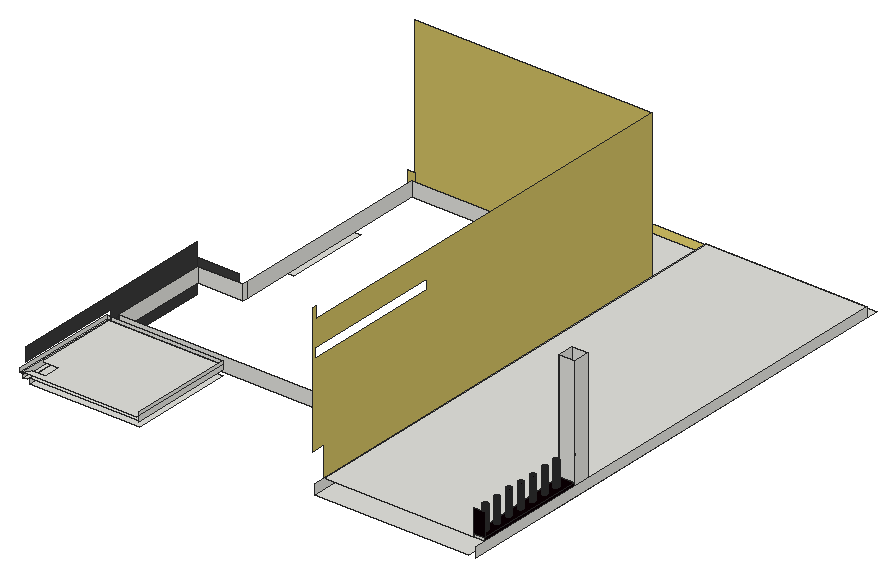
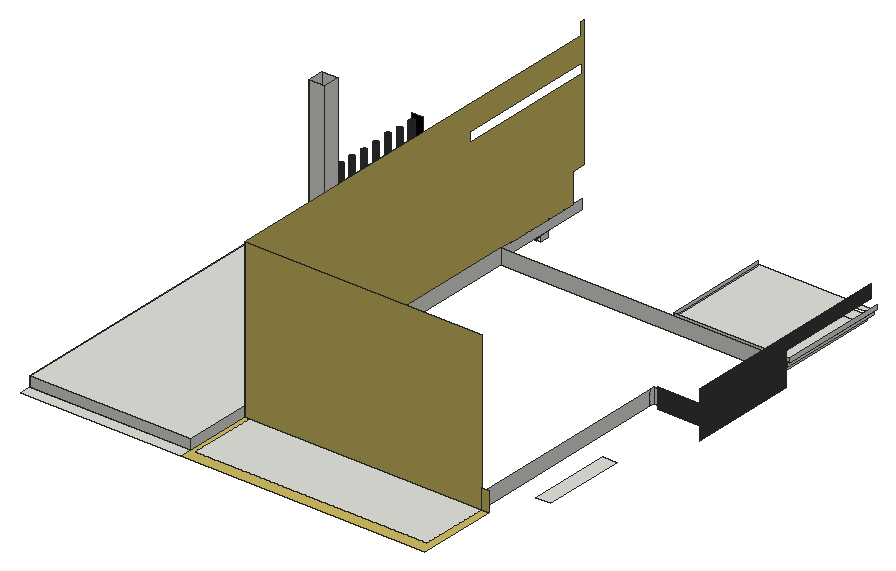
# SketchUp Ruby script. Lengths in inches.
U = 1.inch
M = Sketchup.active_model
def pt(a) = Geom::Point3d.new(a.map { |v| v * U })
def face(e, loops, mat)
  f = e.add_face(loops[0].map { |a| pt(a) })
  loops[1..].each { |l| e.add_face(l.map { |a| pt(a) }).erase! }
  f.material = f.back_material = mat if mat
  f
end
# faces: each face lists its corners as indices into pts; further lists are holes
def faces(e, pts, list, mat = nil) = list.each { |f| face(e, (f[0].is_a?(Array) ? f : [f]).map { |l| l.map { |i| pts[i] } }, mat) }
# xy, xz, yz: faces in a plane at the given z, y or x. An outline is a flat list of corners, or four numbers for a rectangle; further outlines are holes
def ring(l) = l.size == 4 ? [[l[0], l[1]], [l[2], l[1]], [l[2], l[3]], [l[0], l[3]]] : l.each_slice(2).to_a
def flat(e, list, mat, &to3) = list.each { |f| face(e, (f[0].is_a?(Array) ? f : [f]).map { |l| ring(l).map { |u, v| to3.(u, v) } }, mat) }
def xy(e, z, list, mat = nil) = flat(e, list, mat) { |x, y| [x, y, z] }
def xz(e, y, list, mat = nil) = flat(e, list, mat) { |x, z| [x, y, z] }
def yz(e, x, list, mat = nil) = flat(e, list, mat) { |y, z| [x, y, z] }
def lines(e, pts, list) = list.each { |a, b| e.add_line(pt(pts[a]), pt(pts[b])) }
# prism: a flat outline (further loops are holes) pulled along v
def prism(e, loops, v, mat = nil)
  f = face(e, loops, mat); d = Geom::Vector3d.new(v.map { |x| x * U })
  f.pushpull(f.normal.samedirection?(d) ? d.length : -d.length)
end
def box(e, o, s, mat = nil) = prism(e, [[o, [o[0] + s[0], o[1], o[2]], [o[0] + s[0], o[1] + s[1], o[2]], [o[0], o[1] + s[1], o[2]]]], [0, 0, s[2]], mat)
def at(x, y, z, deg = 0) = Geom::Transformation.translation(pt([x, y, z])) * Geom::Transformation.rotation(ORIGIN, Z_AXIS, deg.degrees)
def axes(o, x, y, z) = Geom::Transformation.new([*x, 0, *y, 0, *z, 0, *pt(o).to_a, 1])
def part(name) = M.definitions.add(name)
# library, detail: a bought-in or finely detailed component or shape, given as its bounding box
def library(name, o, s) = part(name).tap { |d| box(d.entities, o, s) }
def detail(e, o, s) = box(e.add_group.entities, o, s)
def put(e, d, t, mat = nil) = e.add_instance(d, t).tap { |i| i.material = mat if mat }
def group(e, t, mat = nil) = e.add_group.tap { |g| g.transformation = t; g.material = mat if mat }.entities
root = M.entities
M.materials.add("[Color D05]").color = [208, 191, 99]
M.materials.add("[Color M07]").color = [58, 58, 58]
M.materials.add("[Metal Seamed]").color = [11, 0, 4]
xy(root,386.54,[[389.45,106.41,450.64,113.66]])
xy(root,386.56,[[384.5,104.22,390.89,113.66],[450.58,104.22,454.38,113.66]])
xy(root,386.84,[[390.89,104.22,450.58,113.66]])
xy(root,392.6,[[55.1875,410.35,72.6875,511.06]])
xy(root,393.87,[[384.5,104.22,454.38,113.66]])
xy(root,408,[[24.25,69.47,158,195.41],[369.3125,70.97,369.3125,113.66,471.3125,113.66,471.3125,195.41,564.5,195.41,564.5,84.18,555.7,84.18,555.7,70.97],[369.3125,113.66,465.3125,119.66],[465.3125,113.66,465.3125,195.41,369.3125,195.41,369.3125,664.97,555.3125,664.97,555.3125,195.41,471.3125,195.41,471.3125,113.66],[369.3125,119.66,465.3125,195.41],
  [555.3125,195.41,564.3125,664.97],[564.3125,195.41,564.5,664.97],[81.6875,582.91,363.3125,665.75],[369.3125,664.97,564.3125,679.25]])
xy(root,408,[[72.6875,582.91,81.6875,582.91,81.6875,665.75,363.3125,665.75,363.3125,582.91,369.3125,582.91,369.3125,679.25,72.6875,679.25]],"[Color D05]")
xy(root,414.75,[[19.4375,65.66,19.4375,195.41,24.25,195.41,24.25,67.28,21.75,67.28,21.75,65.66],[24.25,69.47,158,195.41]])
xy(root,420,[[369.3125,84.66,550.8125,84.66,545.3,221.65,545.3,240.85,564.5,240.85,564.5,664.97,369.3125,664.97],[550.8125,84.66,545.3,221.65,564.5,221.65,564.5,84.66],[545.3,221.65,564.5,240.85]])
xy(root,420.5,[[17.375,63.91,17.375,195.41,19.4375,195.41,19.4375,65.66,21.75,65.66,21.75,63.91],[19.4375,65.66,158,65.66,158,195.41,19.4375,195.41,19.4375,92.83,41.19,92.83,41.19,73.08,24.07,73.08,24.07,70.02,19.4375,70.02]])
xy(root,423.375,[[554.92,94.18,554.11,94.29,553.36,94.6,552.71,95.1,552.21,95.75,551.9,96.5,551.79,97.31,551.9,98.12,552.21,98.87,552.71,99.52,553.36,100.01,554.11,100.33,554.92,100.43,555.73,100.33,556.48,100.01,557.13,99.52,557.625,98.87,557.9375,98.12,558.04,97.31,557.9375,96.5,557.625,95.75,557.13,95.1,556.48,94.6,555.73,94.29],[554.92,130.31,554.11,130.41,553.36,130.73,552.71,131.22,552.21,131.87,551.9,132.625,551.79,133.43,551.9,134.24,552.21,135,552.71,135.64,553.36,136.14,554.11,136.45,554.92,136.56,555.73,136.45,556.48,136.14,557.13,135.64,557.625,135,557.9375,134.24,558.04,133.43,557.9375,132.625,557.625,131.87,557.13,131.22,556.48,130.73,555.73,130.41],[554.92,148.37,554.11,148.48,553.36,148.79,552.71,149.29,552.21,149.93,551.9,150.6875,551.79,151.5,551.9,152.3,552.21,153.06,552.71,153.71,553.36,154.2,554.11,154.51,554.92,154.62,555.73,154.51,556.48,154.2,557.13,153.71,557.625,153.06,557.9375,152.3,558.04,151.5,557.9375,150.6875,557.625,149.93,557.13,149.29,556.48,148.79,555.73,148.48],[554.92,166.43,554.11,166.54,553.36,166.85,552.71,167.35,552.21,168,551.9,168.75,551.79,169.56,551.9,170.37,552.21,171.12,552.71,171.77,553.36,172.26,554.11,172.58,554.92,172.68,555.73,172.58,556.48,172.26,557.13,171.77,557.625,171.12,557.9375,170.37,558.04,169.56,557.9375,168.75,557.625,168,557.13,167.35,556.48,166.85,555.73,166.54],[554.92,184.5,554.11,184.6,553.36,184.91,552.71,185.41,552.21,186.06,551.9,186.8125,551.79,187.62,551.9,188.43,552.21,189.18,552.71,189.83,553.36,190.33,554.11,190.64,554.92,190.75,555.73,190.64,556.48,190.33,557.13,189.83,557.625,189.18,557.9375,188.43,558.04,187.62,557.9375,186.8125,557.625,186.06,557.13,185.41,556.48,184.91,555.73,184.6],
  [554.92,201.87,554.11,201.98,553.36,202.29,552.71,202.79,552.21,203.43,551.9,204.1875,551.79,205,551.9,205.8,552.21,206.56,552.71,207.21,553.36,207.7,554.11,208.01,554.92,208.12,555.73,208.01,556.48,207.7,557.13,207.21,557.625,206.56,557.9375,205.8,558.04,205,557.9375,204.1875,557.625,203.43,557.13,202.79,556.48,202.29,555.73,201.98]])
xy(root,423.375,[[[550.8125,84.66,564.5,84.66,564.5,221.65,545.3,221.65],[554.92,94.18,554.11,94.29,553.36,94.6,552.71,95.1,552.21,95.75,551.9,96.5,551.79,97.31,551.9,98.12,552.21,98.87,552.71,99.52,553.36,100.01,554.11,100.33,554.92,100.43,555.73,100.33,556.48,100.01,557.13,99.52,557.625,98.87,557.9375,98.12,558.04,97.31,557.9375,96.5,557.625,95.75,557.13,95.1,556.48,94.6,555.73,94.29],[554.92,112.25,554.11,112.35,553.36,112.66,552.71,113.16,552.21,113.81,551.9,114.5625,551.79,115.37,551.9,116.18,552.21,116.93,552.71,117.58,553.36,118.08,554.11,118.39,554.92,118.5,555.73,118.39,556.48,118.08,557.13,117.58,557.625,116.93,557.9375,116.18,558.04,115.37,557.9375,114.5625,557.625,113.81,557.13,113.16,556.48,112.66,555.73,112.35],[554.92,130.31,554.11,130.41,553.36,130.73,552.71,131.22,552.21,131.87,551.9,132.625,551.79,133.43,551.9,134.24,552.21,135,552.71,135.64,553.36,136.14,554.11,136.45,554.92,136.56,555.73,136.45,556.48,136.14,557.13,135.64,557.625,135,557.9375,134.24,558.04,133.43,557.9375,132.625,557.625,131.87,557.13,131.22,556.48,130.73,555.73,130.41],[554.92,148.37,554.11,148.48,553.36,148.79,552.71,149.29,552.21,149.93,551.9,150.6875,551.79,151.5,551.9,152.3,552.21,153.06,552.71,153.71,553.36,154.2,554.11,154.51,554.92,154.62,555.73,154.51,556.48,154.2,557.13,153.71,557.625,153.06,557.9375,152.3,558.04,151.5,557.9375,150.6875,557.625,149.93,557.13,149.29,556.48,148.79,555.73,148.48],[554.92,166.43,554.11,166.54,553.36,166.85,552.71,167.35,552.21,168,551.9,168.75,551.79,169.56,551.9,170.37,552.21,171.12,552.71,171.77,553.36,172.26,554.11,172.58,554.92,172.68,555.73,172.58,556.48,172.26,557.13,171.77,557.625,171.12,557.9375,170.37,558.04,169.56,557.9375,168.75,557.625,168,557.13,167.35,556.48,166.85,555.73,166.54],[554.92,184.5,554.11,184.6,553.36,184.91,552.71,185.41,552.21,186.06,551.9,186.8125,551.79,187.62,551.9,188.43,552.21,189.18,552.71,189.83,553.36,190.33,554.11,190.64,554.92,190.75,555.73,190.64,556.48,190.33,557.13,189.83,557.625,189.18,557.9375,188.43,558.04,187.62,557.9375,186.8125,557.625,186.06,557.13,185.41,556.48,184.91,555.73,184.6],[554.92,201.87,554.11,201.98,553.36,202.29,552.71,202.79,552.21,203.43,551.9,204.1875,551.79,205,551.9,205.8,552.21,206.56,552.71,207.21,553.36,207.7,554.11,208.01,554.92,208.12,555.73,208.01,556.48,207.7,557.13,207.21,557.625,206.56,557.9375,205.8,558.04,205,557.9375,204.1875,557.625,203.43,557.13,202.79,556.48,202.29,555.73,201.98]]],"[Metal Seamed]")
xz(root,84.66,[[550.8125,420,564.5,423.375]])
xz(root,84.66,[[550.8125,423.375,564.5,451.5625]],"[Metal Seamed]")
xz(root,104.22,[[384.5,386.56,390.89,386.56,390.89,386.84,450.58,386.84,450.58,386.56,454.38,386.56,454.38,393.87,384.5,393.87]])
xz(root,195.41,[[21.75,408,24.25,414.75],[19.4375,414.75,21.75,420.5],[21.75,414.75,158,420.5],[17.375,420.5,21.75,425],[21.75,420.5,158,425]])
xz(root,201.41,[[26.75,408,363.3125,426]])
xz(root,221.65,[[545.3,420,564.5,423.375],[545.3,423.375,564.5,423.375,564.5,451.5625,563.5625,451.5625,563.5625,456,564.5,456,564.5,555.625,545.3,555.625]])
xz(root,240.85,[[545.3,420,564.5,555.625]])
xz(root,320.85,[[26.75,408,81.6875,426]])
xz(root,326.53,[[21.75,408,72.6875,432]],"[Color M07]")
xz(root,578.04,[[81.6875,408,363.3125,426]])
xz(root,582.91,[[72.6875,408,81.6875,432],[81.6875,408,369.3125,598.25]],"[Color D05]")
xz(root,664.97,[[369.3125,408,564.5,420]])
yz(root,17.375,[[63.91,420.5,195.41,425]])
yz(root,19.4375,[[65.66,414.75,195.41,420.5]])
yz(root,21.75,[[195.41,391.47,326.53,420.03],[195.41,420.03,195.41,432,67.28,432,67.28,448.0625,326.53,448.0625,326.53,420.03]],"[Color M07]")
yz(root,24.25,[[69.47,408,195.41,414.75]])
yz(root,26.75,[[201.41,408,320.85,426]])
yz(root,81.6875,[[320.85,408,326.53,426],[326.53,408,578.04,426]])
yz(root,158,[[67.28,414.75,195.41,420.5],[67.28,420.5,195.41,425]])
yz(root,363.3125,[[201.41,408,578.04,426]])
yz(root,369.3125,[[70.97,408,582.91,420],[582.91,408,664.97,420]])
yz(root,369.3125,[[[84.66,420,582.91,420,582.91,598.25,72.19,598.25,72.19,612.8125,67.28,612.8125,67.28,456,84.66,456],[70.97,555.625,240.85,567.625]]],"[Color D05]")
yz(root,384.5,[[104.22,386.56,113.66,393.87]])
yz(root,390.89,[[104.22,386.56,113.66,386.84]])
yz(root,450.58,[[104.22,386.56,113.66,386.84]])
yz(root,454.38,[[104.22,386.56,113.66,393.87]])
yz(root,545.3,[[221.65,420,240.85,555.625]])
yz(root,564.5,[[70.97,408,664.97,420],[221.65,420,240.85,420,240.85,555.625,221.65,555.625,221.65,456,222.34,456,222.34,451.5625,221.65,451.5625]])
yz(root,564.5,[[84.66,420,221.65,423.375]],"[Metal Seamed]")
p = [[545.3,221.65,420],[550.8125,84.66,420],[550.8125,84.66,423.375],[545.3,221.65,423.375],[554.11,94.29,423.375],[554.92,94.18,423.375],
  [554.92,94.18,451.5625],[554.11,94.29,451.5625],[555.73,94.29,423.375],[555.73,94.29,451.5625],[553.36,94.6,423.375],[553.36,94.6,451.5625],
  [556.48,94.6,423.375],[556.48,94.6,451.5625],[552.71,95.1,423.375],[552.71,95.1,451.5625],[557.13,95.1,423.375],[557.13,95.1,451.5625],
  [552.21,95.75,423.375],[552.21,95.75,451.5625],[557.625,95.75,423.375],[557.625,95.75,451.5625],[551.9,96.5,423.375],[551.9,96.5,451.5625],
  [557.9375,96.5,423.375],[557.9375,96.5,451.5625],[551.79,97.31,423.375],[551.79,97.31,451.5625],[558.04,97.31,423.375],[558.04,97.31,451.5625],
  [551.9,98.12,423.375],[551.9,98.12,451.5625],[557.9375,98.12,423.375],[557.9375,98.12,451.5625],[552.21,98.87,423.375],[552.21,98.87,451.5625],
  [557.625,98.87,423.375],[557.625,98.87,451.5625],[552.71,99.52,423.375],[552.71,99.52,451.5625],[557.13,99.52,423.375],[557.13,99.52,451.5625],
  [553.36,100.01,423.375],[553.36,100.01,451.5625],[556.48,100.01,423.375],[556.48,100.01,451.5625],[554.11,100.33,423.375],[554.11,100.33,451.5625],
  [555.73,100.33,423.375],[555.73,100.33,451.5625],[554.92,100.43,423.375],[554.92,100.43,451.5625],[554.11,112.35,423.375],[554.92,112.25,423.375],
  [554.92,112.25,451.5],[554.11,112.35,451.5],[555.73,112.35,423.375],[555.73,112.35,451.5],[553.36,112.66,423.375],[553.36,112.66,451.5],
  [556.48,112.66,423.375],[556.48,112.66,451.5],[552.71,113.16,423.375],[552.71,113.16,451.5],[557.13,113.16,423.375],[557.13,113.16,451.5],
  [552.21,113.81,423.375],[552.21,113.81,451.5],[557.625,113.81,423.375],[557.625,113.81,451.5],[551.9,114.5625,423.375],[551.9,114.5625,451.5],
  [557.9375,114.5625,423.375],[557.9375,114.5625,451.5],[551.79,115.37,423.375],[551.79,115.37,451.5],[558.04,115.37,423.375],[558.04,115.37,451.5],
  [551.9,116.18,423.375],[551.9,116.18,451.5],[557.9375,116.18,423.375],[557.9375,116.18,451.5],[552.21,116.93,423.375],[552.21,116.93,451.5],
  [557.625,116.93,423.375],[557.625,116.93,451.5],[552.71,117.58,423.375],[552.71,117.58,451.5],[557.13,117.58,423.375],[557.13,117.58,451.5],
  [553.36,118.08,423.375],[553.36,118.08,451.5],[556.48,118.08,423.375],[556.48,118.08,451.5],[554.11,118.39,423.375],[554.11,118.39,451.5],
  [555.73,118.39,423.375],[555.73,118.39,451.5],[554.92,118.5,423.375],[554.92,118.5,451.5],[554.11,130.41,423.375],[554.92,130.31,423.375],
  [554.92,130.31,453.1875],[554.11,130.41,453.1875],[555.73,130.41,423.375],[555.73,130.41,453.1875],[553.36,130.73,423.375],[553.36,130.73,453.1875],
  [556.48,130.73,423.375],[556.48,130.73,453.1875],[552.71,131.22,423.375],[552.71,131.22,453.1875],[557.13,131.22,423.375],[557.13,131.22,453.1875],
  [552.21,131.87,423.375],[552.21,131.87,453.1875],[557.625,131.87,423.375],[557.625,131.87,453.1875],[551.9,132.625,423.375],[551.9,132.625,453.1875],
  [557.9375,132.625,423.375],[557.9375,132.625,453.1875],[551.79,133.43,423.375],[551.79,133.43,453.1875],[558.04,133.43,423.375],[558.04,133.43,453.1875],
  [551.9,134.24,423.375],[551.9,134.24,453.1875],[557.9375,134.24,423.375],[557.9375,134.24,453.1875],[552.21,135,423.375],[552.21,135,453.1875],
  [557.625,135,423.375],[557.625,135,453.1875],[552.71,135.64,423.375],[552.71,135.64,453.1875],[557.13,135.64,423.375],[557.13,135.64,453.1875],
  [553.36,136.14,423.375],[553.36,136.14,453.1875],[556.48,136.14,423.375],[556.48,136.14,453.1875],[554.11,136.45,423.375],[554.11,136.45,453.1875],
  [555.73,136.45,423.375],[555.73,136.45,453.1875],[554.92,136.56,423.375],[554.92,136.56,453.1875],[554.11,148.48,423.375],[554.92,148.37,423.375],
  [554.92,148.37,451.75],[554.11,148.48,451.75],[555.73,148.48,423.375],[555.73,148.48,451.75],[553.36,148.79,423.375],[553.36,148.79,451.75],
  [556.48,148.79,423.375],[556.48,148.79,451.75],[552.71,149.29,423.375],[552.71,149.29,451.75],[557.13,149.29,423.375],[557.13,149.29,451.75],
  [552.21,149.93,423.375],[552.21,149.93,451.75],[557.625,149.93,423.375],[557.625,149.93,451.75],[551.9,150.6875,423.375],[551.9,150.6875,451.75],
  [557.9375,150.6875,423.375],[557.9375,150.6875,451.75],[551.79,151.5,423.375],[551.79,151.5,451.75],[558.04,151.5,423.375],[558.04,151.5,451.75],
  [551.9,152.3,423.375],[551.9,152.3,451.75],[557.9375,152.3,423.375],[557.9375,152.3,451.75],[552.21,153.06,423.375],[552.21,153.06,451.75],
  [557.625,153.06,423.375],[557.625,153.06,451.75],[552.71,153.71,423.375],[552.71,153.71,451.75],[557.13,153.71,423.375],[557.13,153.71,451.75],
  [553.36,154.2,423.375],[553.36,154.2,451.75],[556.48,154.2,423.375],[556.48,154.2,451.75],[554.11,154.51,423.375],[554.11,154.51,451.75],
  [555.73,154.51,423.375],[555.73,154.51,451.75],[554.92,154.62,423.375],[554.92,154.62,451.75],[554.11,166.54,423.375],[554.92,166.43,423.375],
  [554.92,166.43,451.5],[554.11,166.54,451.5],[555.73,166.54,423.375],[555.73,166.54,451.5],[553.36,166.85,423.375],[553.36,166.85,451.5],
  [556.48,166.85,423.375],[556.48,166.85,451.5],[552.71,167.35,423.375],[552.71,167.35,451.5],[557.13,167.35,423.375],[557.13,167.35,451.5],
  [552.21,168,423.375],[552.21,168,451.5],[557.625,168,423.375],[557.625,168,451.5],[551.9,168.75,423.375],[551.9,168.75,451.5],
  [557.9375,168.75,423.375],[557.9375,168.75,451.5],[551.79,169.56,423.375],[551.79,169.56,451.5],[558.04,169.56,423.375],[558.04,169.56,451.5],
  [551.9,170.37,423.375],[551.9,170.37,451.5],[557.9375,170.37,423.375],[557.9375,170.37,451.5],[552.21,171.12,423.375],[552.21,171.12,451.5],
  [557.625,171.12,423.375],[557.625,171.12,451.5],[552.71,171.77,423.375],[552.71,171.77,451.5],[557.13,171.77,423.375],[557.13,171.77,451.5],
  [553.36,172.26,423.375],[553.36,172.26,451.5],[556.48,172.26,423.375],[556.48,172.26,451.5],[554.11,172.58,423.375],[554.11,172.58,451.5],
  [555.73,172.58,423.375],[555.73,172.58,451.5],[554.92,172.68,423.375],[554.92,172.68,451.5],[554.11,184.6,423.375],[554.92,184.5,423.375],
  [554.92,184.5,452.5],[554.11,184.6,452.5],[555.73,184.6,423.375],[555.73,184.6,452.5],[553.36,184.91,423.375],[553.36,184.91,452.5],
  [556.48,184.91,423.375],[556.48,184.91,452.5],[552.71,185.41,423.375],[552.71,185.41,452.5],[557.13,185.41,423.375],[557.13,185.41,452.5],
  [552.21,186.06,423.375],[552.21,186.06,452.5],[557.625,186.06,423.375],[557.625,186.06,452.5],[551.9,186.8125,423.375],[551.9,186.8125,452.5],
  [557.9375,186.8125,423.375],[557.9375,186.8125,452.5],[551.79,187.62,423.375],[551.79,187.62,452.5],[558.04,187.62,423.375],[558.04,187.62,452.5],
  [551.9,188.43,423.375],[551.9,188.43,452.5],[557.9375,188.43,423.375],[557.9375,188.43,452.5],[552.21,189.18,423.375],[552.21,189.18,452.5],
  [557.625,189.18,423.375],[557.625,189.18,452.5],[552.71,189.83,423.375],[552.71,189.83,452.5],[557.13,189.83,423.375],[557.13,189.83,452.5],
  [553.36,190.33,423.375],[553.36,190.33,452.5],[556.48,190.33,423.375],[556.48,190.33,452.5],[554.11,190.64,423.375],[554.11,190.64,452.5],
  [555.73,190.64,423.375],[555.73,190.64,452.5],[554.92,190.75,423.375],[554.92,190.75,452.5],[554.11,201.98,423.375],[554.92,201.87,423.375],
  [554.92,201.87,452.4375],[554.11,201.98,452.4375],[555.73,201.98,423.375],[555.73,201.98,452.4375],[553.36,202.29,423.375],[553.36,202.29,452.4375],
  [556.48,202.29,423.375],[556.48,202.29,452.4375],[552.71,202.79,423.375],[552.71,202.79,452.4375],[557.13,202.79,423.375],[557.13,202.79,452.4375],
  [552.21,203.43,423.375],[552.21,203.43,452.4375],[557.625,203.43,423.375],[557.625,203.43,452.4375],[551.9,204.1875,423.375],[551.9,204.1875,452.4375],
  [557.9375,204.1875,423.375],[557.9375,204.1875,452.4375],[551.79,205,423.375],[551.79,205,452.4375],[558.04,205,423.375],[558.04,205,452.4375],
  [551.9,205.8,423.375],[551.9,205.8,452.4375],[557.9375,205.8,423.375],[557.9375,205.8,452.4375],[552.21,206.56,423.375],[552.21,206.56,452.4375],
  [557.625,206.56,423.375],[557.625,206.56,452.4375],[552.71,207.21,423.375],[552.71,207.21,452.4375],[557.13,207.21,423.375],[557.13,207.21,452.4375],
  [553.36,207.7,423.375],[553.36,207.7,452.4375],[556.48,207.7,423.375],[556.48,207.7,452.4375],[554.11,208.01,423.375],[554.11,208.01,452.4375],
  [555.73,208.01,423.375],[555.73,208.01,452.4375],[554.92,208.12,423.375],[554.92,208.12,452.4375]]
faces(root,p,[[0,1,2,3],[4,5,6,7],[5,8,9,6],[10,4,7,11],[8,12,13,9],[14,10,11,15],[12,16,17,13],[18,14,15,19],
  [16,20,21,17],[22,18,19,23],[20,24,25,21],[26,22,23,27],[24,28,29,25],[30,26,27,31],[28,32,33,29],[34,30,31,35],
  [32,36,37,33],[38,34,35,39],[36,40,41,37],[42,38,39,43],[40,44,45,41],[46,42,43,47],[44,48,49,45],[50,46,47,51],
  [48,50,51,49],[52,53,54,55],[53,56,57,54],[58,52,55,59],[56,60,61,57],[62,58,59,63],[60,64,65,61],[66,62,63,67],
  [64,68,69,65],[70,66,67,71],[68,72,73,69],[74,70,71,75],[72,76,77,73],[78,74,75,79],[76,80,81,77],[82,78,79,83],
  [80,84,85,81],[86,82,83,87],[84,88,89,85],[90,86,87,91],[88,92,93,89],[94,90,91,95],[92,96,97,93],[98,94,95,99],
  [96,98,99,97],[100,101,102,103],[101,104,105,102],[106,100,103,107],[104,108,109,105],[110,106,107,111],[108,112,113,109],[114,110,111,115],
  [112,116,117,113],[118,114,115,119],[116,120,121,117],[122,118,119,123],[120,124,125,121],[126,122,123,127],[124,128,129,125],[130,126,127,131],
  [128,132,133,129],[134,130,131,135],[132,136,137,133],[138,134,135,139],[136,140,141,137],[142,138,139,143],[140,144,145,141],[146,142,143,147],
  [144,146,147,145],[148,149,150,151],[149,152,153,150],[154,148,151,155],[152,156,157,153],[158,154,155,159],[156,160,161,157],[162,158,159,163],
  [160,164,165,161],[166,162,163,167],[164,168,169,165],[170,166,167,171],[168,172,173,169],[174,170,171,175],[172,176,177,173],[178,174,175,179],
  [176,180,181,177],[182,178,179,183],[180,184,185,181],[186,182,183,187],[184,188,189,185],[190,186,187,191],[188,192,193,189],[194,190,191,195],
  [192,194,195,193],[196,197,198,199],[197,200,201,198],[202,196,199,203],[200,204,205,201],[206,202,203,207],[204,208,209,205],[210,206,207,211],
  [208,212,213,209],[214,210,211,215],[212,216,217,213],[218,214,215,219],[216,220,221,217],[222,218,219,223],[220,224,225,221],[226,222,223,227],
  [224,228,229,225],[230,226,227,231],[228,232,233,229],[234,230,231,235],[232,236,237,233],[238,234,235,239],[236,240,241,237],[242,238,239,243],
  [240,242,243,241],[244,245,246,247],[245,248,249,246],[250,244,247,251],[248,252,253,249],[254,250,251,255],[252,256,257,253],[258,254,255,259],
  [256,260,261,257],[262,258,259,263],[260,264,265,261],[266,262,263,267],[264,268,269,265],[270,266,267,271],[268,272,273,269],[274,270,271,275],
  [272,276,277,273],[278,274,275,279],[276,280,281,277],[282,278,279,283],[280,284,285,281],[286,282,283,287],[284,288,289,285],[290,286,287,291],
  [288,290,291,289],[292,293,294,295],[293,296,297,294],[298,292,295,299],[296,300,301,297],[302,298,299,303],[300,304,305,301],[306,302,303,307],
  [304,308,309,305],[310,306,307,311],[308,312,313,309],[314,310,311,315],[312,316,317,313],[318,314,315,319],[316,320,321,317],[322,318,319,323],
  [320,324,325,321],[326,322,323,327],[324,328,329,325],[330,326,327,331],[328,332,333,329],[334,330,331,335],[332,336,337,333],[338,334,335,339],
  [336,338,339,337]],"[Metal Seamed]")
